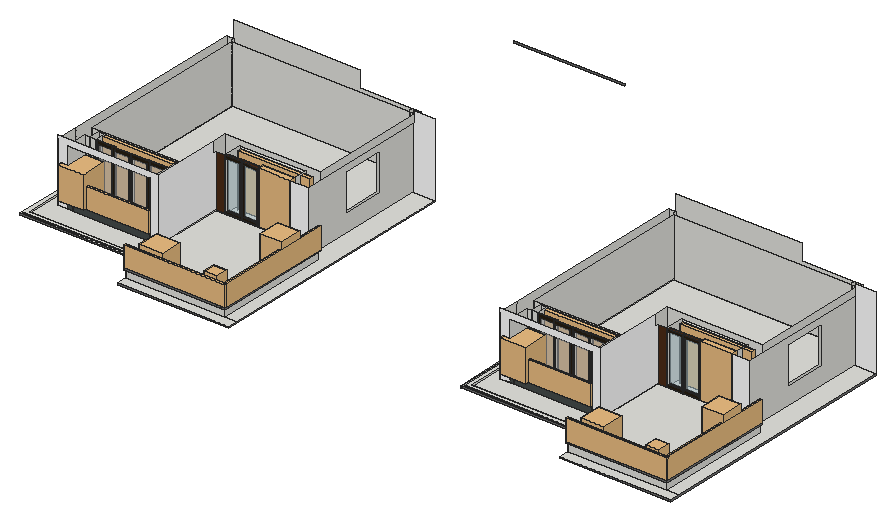
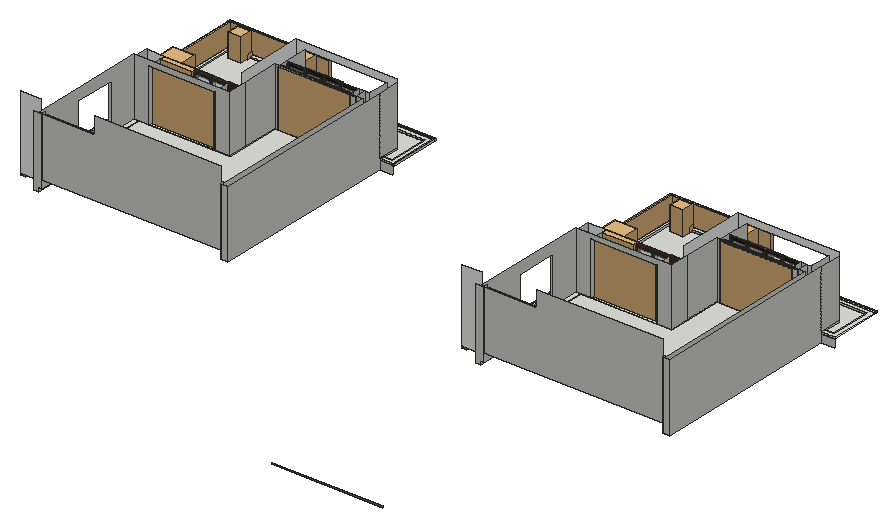
# SketchUp Ruby script. Lengths in inches.
U = 1.inch
M = Sketchup.active_model
def pt(a) = Geom::Point3d.new(a.map { |v| v * U })
def face(e, loops, mat)
  f = e.add_face(loops[0].map { |a| pt(a) })
  loops[1..].each { |l| e.add_face(l.map { |a| pt(a) }).erase! }
  f.material = f.back_material = mat if mat
  f
end
# faces: each face lists its corners as indices into pts; further lists are holes
def faces(e, pts, list, mat = nil) = list.each { |f| face(e, (f[0].is_a?(Array) ? f : [f]).map { |l| l.map { |i| pts[i] } }, mat) }
# xy, xz, yz: faces in a plane at the given z, y or x. An outline is a flat list of corners, or four numbers for a rectangle; further outlines are holes
def ring(l) = l.size == 4 ? [[l[0], l[1]], [l[2], l[1]], [l[2], l[3]], [l[0], l[3]]] : l.each_slice(2).to_a
def flat(e, list, mat, &to3) = list.each { |f| face(e, (f[0].is_a?(Array) ? f : [f]).map { |l| ring(l).map { |u, v| to3.(u, v) } }, mat) }
def xy(e, z, list, mat = nil) = flat(e, list, mat) { |x, y| [x, y, z] }
def xz(e, y, list, mat = nil) = flat(e, list, mat) { |x, z| [x, y, z] }
def yz(e, x, list, mat = nil) = flat(e, list, mat) { |y, z| [x, y, z] }
def lines(e, pts, list) = list.each { |a, b| e.add_line(pt(pts[a]), pt(pts[b])) }
# prism: a flat outline (further loops are holes) pulled along v
def prism(e, loops, v, mat = nil)
  f = face(e, loops, mat); d = Geom::Vector3d.new(v.map { |x| x * U })
  f.pushpull(f.normal.samedirection?(d) ? d.length : -d.length)
end
def box(e, o, s, mat = nil) = prism(e, [[o, [o[0] + s[0], o[1], o[2]], [o[0] + s[0], o[1] + s[1], o[2]], [o[0], o[1] + s[1], o[2]]]], [0, 0, s[2]], mat)
def at(x, y, z, deg = 0) = Geom::Transformation.translation(pt([x, y, z])) * Geom::Transformation.rotation(ORIGIN, Z_AXIS, deg.degrees)
def axes(o, x, y, z) = Geom::Transformation.new([*x, 0, *y, 0, *z, 0, *pt(o).to_a, 1])
def part(name) = M.definitions.add(name)
# library, detail: a bought-in or finely detailed component or shape, given as its bounding box
def library(name, o, s) = part(name).tap { |d| box(d.entities, o, s) }
def detail(e, o, s) = box(e.add_group.entities, o, s)
def put(e, d, t, mat = nil) = e.add_instance(d, t).tap { |i| i.material = mat if mat }
def group(e, t, mat = nil) = e.add_group.tap { |g| g.transformation = t; g.material = mat if mat }.entities
root = M.entities
M.materials.add("[Color M00]").color = [255, 255, 255]
M.materials.add("[Color M05]").color = [114, 114, 114]
M.materials.add("[Slate]").color = [70, 76, 75]
M.materials.add("[Translucent Glass Gray]2").color = [201, 201, 201]
M.materials["[Translucent Glass Gray]2"].alpha = 0.5
M.materials.add("[Translucent Glass Safety]").color = [204, 235, 244]
M.materials["[Translucent Glass Safety]"].alpha = 0.5
M.materials.add("[Wood Veneer 01]").color = [76, 44, 23]
M.materials.add("oak swatch").color = [40, 31, 19]
c1 = library("Glass Railing",[0,0,0],[139.5,4.76,42])
c2 = library("Plant",[0,0,0],[12.59,12.59,14.16])
c3 = library("plant1",[-367.84,-375.82,-125.45],[750.59,696.16,1346.74])
c4 = part("skp4FF")
put(c4.entities,c3,at(0,0,0))
c5 = library("Flora+17",[-57.52,158.6,-38.64],[66.99,62.88,77.28])
c6 = library("plant (1)",[-35.72,-28.42,0],[66.31,67.39,84.38])
c7 = part("Group\#6")
box(c7.entities,[0,0,0],[1.77,4.72,80.31],"oak swatch")
c8 = part("Exterior Sliding Doors")
xy(c8.entities,0,[[1.77,33.07,3.54,70.87],[1.77,70.87,3.54,108.66]])
xy(c8.entities,0,[[0,0,1.77,33.07],[0,108.66,1.77,141.73]],"oak swatch")
xy(c8.entities,4.72,[[0,4.72,1.77,33.07],[1.77,37.8,3.54,66.14],[1.77,75.88,3.54,103.9375],[0,108.66,1.77,137.01]],"oak swatch")
xy(c8.entities,75.59,[[1.77,37.8,3.54,66.14],[1.77,75.88,3.54,103.9375]])
xy(c8.entities,75.59,[[0,4.72,1.77,33.07],[0,108.66,1.77,137.01]],"oak swatch")
xy(c8.entities,80.31,[[0,0,1.77,33.07],[1.77,33.07,3.54,70.87],[1.77,70.87,3.54,108.66],[0,108.66,1.77,141.73]],"oak swatch")
xz(c8.entities,0,[[0,0,1.77,80.31]],"oak swatch")
xz(c8.entities,4.72,[[0,4.72,1.77,75.59]],"oak swatch")
xz(c8.entities,33.07,[[0,0,1.77,4.72],[1.77,0,3.54,80.31],[0,75.59,1.77,80.31]],"oak swatch")
xz(c8.entities,37.8,[[1.77,4.72,3.54,75.59]])
xz(c8.entities,66.14,[[1.77,4.72,3.54,75.59]],"oak swatch")
xz(c8.entities,70.87,[[1.77,0,3.54,80.31]])
xz(c8.entities,75.88,[[1.77,4.72,3.54,75.59]])
xz(c8.entities,103.9375,[[1.77,4.72,3.54,75.59]],"oak swatch")
xz(c8.entities,108.66,[[1.77,4.72,3.54,75.59]])
xz(c8.entities,108.66,[[0,0,3.54,4.72],[0,75.59,3.54,80.31]],"oak swatch")
xz(c8.entities,137.01,[[0,4.72,1.77,75.59]],"oak swatch")
xz(c8.entities,141.73,[[0,0,1.77,80.31]],"oak swatch")
yz(c8.entities,0,[[0,0,33.07,0,33.07,4.72,4.72,4.72,4.72,75.59,33.07,75.59,33.07,80.31,0,80.31],[108.66,0,141.73,0,141.73,80.31,108.66,80.31,108.66,75.59,137.01,75.59,137.01,4.72,108.66,4.72]],"oak swatch")
yz(c8.entities,1.77,[[4.72,4.72,33.07,75.59],[37.8,4.72,66.14,75.59],[75.88,4.72,103.9375,75.59],[108.66,4.72,137.01,75.59]],"[Translucent Glass Gray]2")
yz(c8.entities,1.77,[[0,0,33.07,0,33.07,4.72,4.72,4.72,4.72,75.59,33.07,75.59,33.07,80.31,0,80.31],[[33.07,0,70.87,80.31],[37.8,4.72,66.14,75.59]],[[70.87,0,141.73,80.31],[108.66,4.72,137.01,75.59],[75.88,4.72,103.9375,75.59]]],"oak swatch")
yz(c8.entities,3.54,[[[33.07,0,70.87,80.31],[37.8,4.72,66.14,75.59]],[[70.87,0,108.66,80.31],[75.88,4.72,103.9375,75.59]]],"oak swatch")
put(c8.entities,c7,at(0,33.07,0))
put(c8.entities,c7,at(0,103.9375,0))
c9 = library("Group\#21",[-0.5,-0.5,-0.1],[115.36,88.99,0.2])
c10 = library("Curtains",[0,0,0],[121.73,8.19,117.22])
c11 = part("Group\#4")
g1 = group(c11.entities,at(0,0,0))
xy(g1,0,[[0,0,6,48]],"[Wood Veneer 01]")
xy(g1,4,[[0,4,1.8125,44],[1.8125,4,6,44]])
xy(g1,80,[[0,4,1.8125,44],[1.8125,4,6,44]])
xy(g1,84,[[0,0,6,48]],"[Wood Veneer 01]")
xz(g1,0,[[0,0,6,84]],"[Wood Veneer 01]")
xz(g1,4,[[0,4,1.8125,80],[1.8125,4,6,80]])
xz(g1,44,[[0,4,1.8125,80],[1.8125,4,6,80]])
xz(g1,48,[[0,0,6,84]],"[Wood Veneer 01]")
yz(g1,0,[[[0,0,48,84],[4,4,44,80]]],"[Wood Veneer 01]")
yz(g1,1.8125,[[4,4,44,80]],"[Translucent Glass Safety]")
yz(g1,6,[[[0,0,48,84],[4,4,44,80]]],"oak swatch")
g2 = group(c11.entities,at(0,48,0),"oak swatch")
xy(g2,0,[[0,0,6,48]],"[Wood Veneer 01]")
xy(g2,4,[[0,4,1.8125,44],[1.8125,4,6,44]])
xy(g2,80,[[0,4,1.8125,44],[1.8125,4,6,44]])
xy(g2,84,[[0,0,6,48]],"[Wood Veneer 01]")
xz(g2,0,[[0,0,6,84]],"[Wood Veneer 01]")
xz(g2,4,[[0,4,1.8125,80],[1.8125,4,6,80]])
xz(g2,44,[[0,4,1.8125,80],[1.8125,4,6,80]])
xz(g2,48,[[0,0,6,84]],"[Wood Veneer 01]")
yz(g2,0,[[[0,0,48,84],[4,4,44,80]]],"[Wood Veneer 01]")
yz(g2,1.8125,[[4,4,44,80]],"[Translucent Glass Safety]")
yz(g2,6,[[[0,0,48,84],[4,4,44,80]]],"oak swatch")
c12 = library("modern+door",[0,0,0],[59.06,11.8125,86.61])
xy(root,119.75,[[2097.23,636.6875,2269.48,636.6875,2269.48,735.75,2276.89,735.75,2276.89,747.5625,2456.54,747.5625,2456.54,1019,2447.32,1019,2447.32,811.54,2440.84,811.54,2440.84,774.3125,2266.54,774.3125,2266.54,645.91,2097.23,645.91],[2989.82,636.6875,3162.07,636.6875,3162.07,735.75,3169.48,735.75,3169.48,747.5625,3349.13,747.5625,3349.13,1019,3339.91,1019,3339.91,811.54,3333.43,811.54,3333.43,774.3125,3159.13,774.3125,3159.13,645.91,2989.82,645.91]])
xy(root,122.875,[[2276.89,479.5,2500.29,488.8125],[3169.48,479.5,3392.88,488.8125],[2489.98,488.8125,2500.29,999.35],[3382.57,488.8125,3392.88,999.35]],"[Color M05]")
xy(root,126,[[2276.89,479.5,2500.29,499.9375],[3169.48,479.5,3392.88,499.9375],[2276.89,499.9375,2475.98,536.1875],[2475.98,499.9375,2500.29,499.9375,2500.29,999.35,2456.54,999.35,2456.54,735.75,2475.98,735.75],[3169.48,499.9375,3368.57,536.1875],
  [3368.57,499.9375,3392.88,499.9375,3392.88,999.35,3349.13,999.35,3349.13,735.75,3368.57,735.75],[2276.89,536.1875,2475.98,636.6875],[3169.48,536.1875,3368.57,636.6875],[2064.92,636.6875,2064.92,1019,2079.65,1019,2079.65,660.21,2097.23,660.21,2097.23,636.6875],[2276.89,636.6875,2475.98,735.75],
  [2957.51,636.6875,2957.51,1019,2972.24,1019,2972.24,660.21,2989.82,660.21,2989.82,636.6875],[3169.48,636.6875,3368.57,735.75],[2097.23,645.91,2097.23,660.21,2256.86,660.21,2256.86,774.3125,2266.54,774.3125,2266.54,645.91],[2989.82,645.91,2989.82,660.21,3149.44,660.21,3149.44,774.3125,3159.13,774.3125,3159.13,645.91],[2276.89,735.75,2456.54,747.5625],
  [3169.48,735.75,3349.13,747.5625],[2440.84,811.54,2447.32,1019],[3333.43,811.54,3339.91,1019]])
xy(root,142.875,[[2276.89,495.25,2475.98,499.9375],[2475.98,495.25,2480.67,499.9375],[3169.48,495.25,3368.57,499.9375],[3368.57,495.25,3373.26,499.9375],[2276.89,499.9375,2276.89,536.1875,2037.92,536.1875,2037.92,636.6875,2064.92,636.6875,2064.92,628.3125,2046.17,628.3125,2046.17,544.8125,2283.23,544.8125,2283.23,507.75,2469.67,507.75,2469.67,721.95,2456.54,721.95,2456.54,735.75,2475.98,735.75,2475.98,499.9375],
  [2475.98,499.9375,2480.67,735.75],[3169.48,499.9375,3169.48,536.1875,2930.51,536.1875,2930.51,636.6875,2957.51,636.6875,2957.51,628.3125,2938.76,628.3125,2938.76,544.8125,3175.82,544.8125,3175.82,507.75,3362.26,507.75,3362.26,721.95,3349.13,721.95,3349.13,735.75,3368.57,735.75,3368.57,499.9375],[3368.57,499.9375,3373.26,735.75],[2283.23,507.75,2469.67,507.75,2469.67,721.95,2456.54,721.95,2456.54,735.75,2269.48,735.75,2269.48,592.75,2064.92,592.75,2064.92,628.3125,2046.17,628.3125,2046.17,544.8125,2283.23,544.8125],[3175.82,507.75,3362.26,507.75,3362.26,721.95,3349.13,721.95,3349.13,735.75,3162.07,735.75,3162.07,592.75,2957.51,592.75,2957.51,628.3125,2938.76,628.3125,2938.76,544.8125,3175.82,544.8125],
  [2037.92,531.5,2276.89,536.1875],[2927.19,531.5,2930.51,536.1875],[2930.51,531.5,3169.48,536.1875],[2927.19,536.1875,2930.32,636.6875],[2930.32,536.1875,2930.51,636.6875],
  [2064.92,592.75,2094.14,592.75,2094.14,604.1,2084.76,604.1,2084.76,636.6875,2064.92,636.6875],[2251.32,592.75,2269.48,636.6875],[2957.51,592.75,2986.73,592.75,2986.73,604.1,2977.35,604.1,2977.35,636.6875,2957.51,636.6875],[3143.91,592.75,3162.07,636.6875],[2084.76,604.1,2251.32,636.6875],
  [2977.35,604.1,3143.91,636.6875],[2094.14,636.6875,2106.51,660.21],[2106.51,636.6875,2251.32,660.21],[2986.73,636.6875,2999.1,660.21],[2999.1,636.6875,3143.91,660.21],
  [2079.65,660.21,2256.86,660.21,2256.86,774.3125,2440.84,774.3125,2440.84,1012.63,2079.65,1012.63],[2972.24,660.21,3149.44,660.21,3149.44,774.3125,3333.43,774.3125,3333.43,1012.63,2972.24,1012.63],[2287.52,735.75,2419.84,774.3125],[3180.11,735.75,3312.43,774.3125],[2440.84,774.3125,2450.84,1012.63],
  [3333.43,774.3125,3343.43,1012.63],[2079.65,1012.63,2440.84,1019],[2972.24,1012.63,3333.43,1019]])
xy(root,146.125,[[2276.89,495.25,2480.67,495.25,2480.67,735.75,2475.98,735.75,2475.98,499.9375,2276.89,499.9375],[3169.48,495.25,3373.26,495.25,3373.26,735.75,3368.57,735.75,3368.57,499.9375,3169.48,499.9375],[2276.89,499.9375,2475.98,499.9375,2475.98,735.75,2456.54,735.75,2456.54,721.95,2469.67,721.95,2469.67,507.75,2283.23,507.75,2283.23,544.8125,2046.17,544.8125,2046.17,628.3125,2064.92,628.3125,2064.92,636.6875,2037.92,636.6875,2037.92,536.1875,2276.89,536.1875],[3169.48,499.9375,3368.57,499.9375,3368.57,735.75,3349.13,735.75,3349.13,721.95,3362.26,721.95,3362.26,507.75,3175.82,507.75,3175.82,544.8125,2938.76,544.8125,2938.76,628.3125,2957.51,628.3125,2957.51,636.6875,2930.51,636.6875,2930.51,536.1875,3169.48,536.1875],[2037.92,531.5,2276.89,536.1875],
  [2927.19,531.5,2930.51,536.1875],[2930.51,531.5,3169.48,536.1875],[2927.19,536.1875,2930.32,636.6875],[2930.32,536.1875,2930.51,636.6875]])
xy(root,156.6875,[[2084.76,592.75,2094.14,604.1],[2094.14,592.75,2251.32,604.1],[2977.35,592.75,2986.73,604.1],[2986.73,592.75,3143.91,604.1]],"[Slate]")
xz(root,479.5,[[2276.89,122.875,2500.29,126],[3169.48,122.875,3392.88,126]],"[Color M05]")
xz(root,495.25,[[2276.89,142.875,2480.67,146.125],[3169.48,142.875,3373.26,146.125]],"[Color M05]")
xz(root,499.9375,[[2276.89,126,2475.98,142.875],[3169.48,126,3368.57,142.875],[2276.89,142.875,2475.98,146.125],[3169.48,142.875,3368.57,146.125]])
xz(root,507.75,[[2283.23,142.875,2469.67,146.125],[3175.82,142.875,3362.26,146.125]])
xz(root,531.5,[[2927.19,142.875,2930.51,146.125]])
xz(root,531.5,[[2037.92,142.875,2276.89,146.125],[2930.51,142.875,3169.48,146.125]],"[Color M05]")
xz(root,536.1875,[[2037.92,142.875,2276.89,146.125],[2927.19,142.875,2930.32,146.125],[2930.32,142.875,2930.51,146.125],[2930.51,142.875,3169.48,146.125]])
xz(root,544.8125,[[2046.17,142.875,2283.23,146.125],[2938.76,142.875,3175.82,146.125]])
xz(root,592.75,[[2064.92,142.875,2084.76,142.875,2084.76,257.1875,2251.32,257.1875,2251.32,142.875,2269.48,142.875,2269.48,270.375,2064.92,270.375],[2957.51,142.875,2977.35,142.875,2977.35,257.1875,3143.91,257.1875,3143.91,142.875,3162.07,142.875,3162.07,270.375,2957.51,270.375]],"[Color M00]")
xz(root,592.75,[[2084.76,142.875,2094.14,156.6875],[2094.14,142.875,2251.32,156.6875],[2977.35,142.875,2986.73,156.6875],[2986.73,142.875,3143.91,156.6875]],"[Slate]")
xz(root,604.1,[[2084.76,142.875,2094.14,156.6875],[2094.14,142.875,2251.32,156.6875],[2977.35,142.875,2986.73,156.6875],[2986.73,142.875,3143.91,156.6875]])
xz(root,628.3125,[[2046.17,142.875,2064.92,146.125],[2938.76,142.875,2957.51,146.125]])
xz(root,636.6875,[[2097.23,119.75,2269.48,119.75,2269.48,142.875,2064.92,142.875,2064.92,126,2097.23,126],[2989.82,119.75,3162.07,119.75,3162.07,142.875,2957.51,142.875,2957.51,126,2989.82,126],[2037.92,126,2064.92,142.875],[2930.51,126,2957.51,142.875],[2037.92,142.875,2064.92,146.125],
  [2084.76,142.875,2094.14,257.1875],[2094.14,142.875,2106.51,257.1875],[2927.19,142.875,2930.32,146.125],[2930.32,142.875,2930.51,146.125],[2930.51,142.875,2957.51,146.125],
  [2977.35,142.875,2986.73,257.1875],[2986.73,142.875,2999.1,257.1875]])
xz(root,645.91,[[2097.23,119.75,2266.54,126],[2989.82,119.75,3159.13,126]])
xz(root,660.21,[[2079.65,126,2256.86,142.875],[2972.24,126,3149.44,142.875],[2079.65,142.875,2079.65,259.3125,2256.86,259.3125,2256.86,142.875,2251.32,142.875,2251.32,257.1875,2094.14,257.1875,2094.14,142.875],[2094.14,142.875,2106.51,257.1875],[2972.24,142.875,2972.24,259.3125,3149.44,259.3125,3149.44,142.875,3143.91,142.875,3143.91,257.1875,2986.73,257.1875,2986.73,142.875],
  [2986.73,142.875,2999.1,257.1875]])
xz(root,721.95,[[2456.54,142.875,2469.67,146.125],[3349.13,142.875,3362.26,146.125]])
xz(root,735.75,[[2269.48,119.75,2276.89,119.75,2276.89,126,2456.54,126,2456.54,142.875,2269.48,142.875],[3162.07,119.75,3169.48,119.75,3169.48,126,3349.13,126,3349.13,142.875,3162.07,142.875],[2456.54,126,2475.98,142.875],[3349.13,126,3368.57,142.875],[2456.54,142.875,2475.98,146.125],
  [2475.98,142.875,2480.67,146.125],[3349.13,142.875,3368.57,146.125],[3368.57,142.875,3373.26,146.125]])
xz(root,735.75,[[2419.84,142.875,2456.54,249.4375],[3312.43,142.875,3349.13,249.4375]],"[Color M00]")
xz(root,735.75,[[2269.48,142.875,2287.52,249.4375],[3162.07,142.875,3180.11,249.4375]],"[Wood Veneer 01]")
xz(root,747.5625,[[2276.89,119.75,2456.54,126],[3169.48,119.75,3349.13,126]])
xz(root,774.3125,[[2266.54,119.75,2440.84,119.75,2440.84,142.875,2256.86,142.875,2256.86,126,2266.54,126],[3159.13,119.75,3333.43,119.75,3333.43,142.875,3149.44,142.875,3149.44,126,3159.13,126],[2256.86,142.875,2256.86,259.3125,2450.84,259.3125,2450.84,142.875,2419.84,142.875,2419.84,249.4375,2287.52,249.4375,2287.52,142.875],[3149.44,142.875,3149.44,259.3125,3343.43,259.3125,3343.43,142.875,3312.43,142.875,3312.43,249.4375,3180.11,249.4375,3180.11,142.875]])
xz(root,811.54,[[2440.84,119.75,2447.32,126],[3333.43,119.75,3339.91,126]])
xz(root,999.35,[[2456.54,126,2500.29,126,2500.29,274.0625,2459.67,274.0625,2459.67,249.4375,2456.54,249.4375],[3349.13,126,3392.88,126,3392.88,274.0625,3352.26,274.0625,3352.26,249.4375,3349.13,249.4375]],"[Color M00]")
xz(root,1012.63,[[2079.65,142.875,2440.84,259.3125],[2440.84,142.875,2450.84,259.3125],[2972.24,142.875,3333.43,259.3125],[3333.43,142.875,3343.43,259.3125]])
xz(root,1019,[[2447.32,119.75,2447.32,126,2440.84,126,2440.84,262.875,2456.54,262.875,2456.54,119.75],[3339.91,119.75,3339.91,126,3333.43,126,3333.43,262.875,3349.13,262.875,3349.13,119.75],[2064.92,126,2079.65,262.875],[2957.51,126,2972.24,262.875],[2079.65,142.875,2079.65,295.8125,2333.29,295.8125,2333.29,262.875,2440.84,262.875,2440.84,142.875],
  [2972.24,142.875,2972.24,295.8125,3225.88,295.8125,3225.88,262.875,3333.43,262.875,3333.43,142.875]])
xz(root,1478.85,[[2276.89,122.875,2500.29,126]],"[Color M05]")
yz(root,2046.17,[[544.8125,142.875,628.3125,146.125]])
yz(root,2064.92,[[636.6875,126,1019,262.875],[592.75,142.875,628.3125,146.125],[628.3125,142.875,636.6875,146.125],[592.75,146.125,636.6875,262.875]])
yz(root,2079.65,[[660.21,126,1019,142.875],[660.21,142.875,1012.63,259.3125],[1012.63,142.875,1019,262.875]])
yz(root,2084.76,[[604.1,142.875,636.6875,142.875,636.6875,257.1875,592.75,257.1875,592.75,156.6875,604.1,156.6875]])
yz(root,2094.14,[[592.75,142.875,604.1,156.6875],[636.6875,142.875,660.21,257.1875]])
yz(root,2097.23,[[636.6875,119.75,645.91,126]])
yz(root,2106.51,[[636.6875,142.875,660.21,257.1875]])
yz(root,2251.32,[[592.75,142.875,604.1,156.6875],[604.1,142.875,604.1,156.6875,592.75,156.6875,592.75,257.1875,636.6875,257.1875,636.6875,142.875],[636.6875,142.875,660.21,257.1875]])
yz(root,2256.86,[[660.21,126,735.75,142.875],[735.75,126,774.3125,142.875],[660.21,142.875,735.75,259.3125],[735.75,142.875,774.3125,259.3125]])
yz(root,2266.54,[[645.91,119.75,774.3125,126]])
yz(root,2269.48,[[636.6875,119.75,735.75,142.875]])
yz(root,2269.48,[[592.75,142.875,735.75,142.875,735.75,249.4375,728.9375,249.4375,728.9375,270.375,592.75,270.375]],"[Color M00]")
yz(root,2276.89,[[735.75,119.75,747.5625,126],[499.9375,126,536.1875,142.875],[495.25,142.875,499.9375,146.125],[499.9375,142.875,531.5,146.125],[531.5,142.875,536.1875,146.125]])
yz(root,2283.23,[[507.75,142.875,544.8125,146.125]])
yz(root,2287.52,[[735.75,142.875,774.3125,249.4375]])
yz(root,2419.84,[[735.75,142.875,774.3125,249.4375]])
yz(root,2440.84,[[774.3125,119.75,811.54,119.75,811.54,126,1019,126,1019,142.875,774.3125,142.875],[1012.63,142.875,1019,262.875]])
yz(root,2447.32,[[811.54,119.75,1019,126]])
yz(root,2450.84,[[[774.3125,142.875,1012.63,259.3125],[831.26,160.58,916.82,236.83]]])
yz(root,2456.54,[[[735.75,126,999.35,249.4375],[831.26,160.58,916.82,236.83]],[721.95,142.875,735.75,146.125]])
yz(root,2469.67,[[507.75,142.875,721.95,146.125]])
yz(root,2475.98,[[499.9375,126,735.75,142.875],[499.9375,142.875,735.75,146.125]])
yz(root,2480.67,[[495.25,142.875,735.75,146.125]],"[Color M05]")
yz(root,2500.29,[[479.5,122.875,999.35,126]],"[Color M05]")
yz(root,2927.19,[[531.5,142.875,536.1875,146.125],[536.1875,142.875,636.6875,146.125]])
yz(root,2930.32,[[536.1875,142.875,636.6875,146.125]])
yz(root,2930.51,[[531.5,142.875,536.1875,146.125],[536.1875,142.875,636.6875,146.125]])
yz(root,2938.76,[[544.8125,142.875,628.3125,146.125]])
yz(root,2957.51,[[636.6875,126,1019,262.875],[592.75,142.875,628.3125,146.125],[628.3125,142.875,636.6875,146.125],[592.75,146.125,636.6875,262.875]])
yz(root,2972.24,[[660.21,126,1019,142.875],[660.21,142.875,1012.63,259.3125],[1012.63,142.875,1019,262.875]])
yz(root,2977.35,[[604.1,142.875,636.6875,142.875,636.6875,257.1875,592.75,257.1875,592.75,156.6875,604.1,156.6875]])
yz(root,2986.73,[[592.75,142.875,604.1,156.6875],[636.6875,142.875,660.21,257.1875]])
yz(root,2989.82,[[636.6875,119.75,645.91,126]])
yz(root,2999.1,[[636.6875,142.875,660.21,257.1875]])
yz(root,3143.91,[[592.75,142.875,604.1,156.6875],[604.1,142.875,604.1,156.6875,592.75,156.6875,592.75,257.1875,636.6875,257.1875,636.6875,142.875],[636.6875,142.875,660.21,257.1875]])
yz(root,3149.44,[[660.21,126,735.75,142.875],[735.75,126,774.3125,142.875],[660.21,142.875,735.75,259.3125],[735.75,142.875,774.3125,259.3125]])
yz(root,3159.13,[[645.91,119.75,774.3125,126]])
yz(root,3162.07,[[636.6875,119.75,735.75,142.875]])
yz(root,3162.07,[[592.75,142.875,735.75,142.875,735.75,249.4375,728.9375,249.4375,728.9375,270.375,592.75,270.375]],"[Color M00]")
yz(root,3169.48,[[735.75,119.75,747.5625,126],[499.9375,126,536.1875,142.875],[495.25,142.875,499.9375,146.125],[499.9375,142.875,531.5,146.125],[531.5,142.875,536.1875,146.125]])
yz(root,3175.82,[[507.75,142.875,544.8125,146.125]])
yz(root,3180.11,[[735.75,142.875,774.3125,249.4375]])
yz(root,3312.43,[[735.75,142.875,774.3125,249.4375]])
yz(root,3333.43,[[774.3125,119.75,811.54,119.75,811.54,126,1019,126,1019,142.875,774.3125,142.875],[1012.63,142.875,1019,262.875]])
yz(root,3339.91,[[811.54,119.75,1019,126]])
yz(root,3343.43,[[[774.3125,142.875,1012.63,259.3125],[831.26,160.58,916.82,236.83]]])
yz(root,3349.13,[[[735.75,126,999.35,249.4375],[831.26,160.58,916.82,236.83]],[721.95,142.875,735.75,146.125]])
yz(root,3362.26,[[507.75,142.875,721.95,146.125]])
yz(root,3368.57,[[499.9375,126,735.75,142.875],[499.9375,142.875,735.75,146.125]])
yz(root,3373.26,[[495.25,142.875,735.75,146.125]],"[Color M05]")
yz(root,3392.88,[[479.5,122.875,999.35,126]],"[Color M05]")
put(root,c1,axes([3169.59,495.25,146.125],[1.46,0,0],[0,1,0],[0,0,1]))
put(root,c1,axes([2277,495.25,146.125],[1.46,0,0],[0,1,0],[0,0,1]))
put(root,c2,axes([3322.12,504.29,142.875],[0.7,0,0],[0,0.7,0],[0,0,0.7]))
put(root,c2,axes([2429.53,504.29,142.875],[0.7,0,0],[0,0.7,0],[0,0,0.7]))
put(root,c4,axes([3335.6,518.07,147.31],[0.03534,0,0],[0,0.03534,0],[0,0,0.03534]))
put(root,c4,axes([2443.01,518.07,147.31],[0.03534,0,0],[0,0.03534,0],[0,0,0.03534]))
put(root,c2,axes([3186.16,515.77,142.875],[0.7,0,0],[0,0.7,0],[0,0,0.7]))
put(root,c2,axes([2293.57,515.77,142.875],[0.7,0,0],[0,0.7,0],[0,0,0.7]))
put(root,c5,axes([3232.35,392.03,165.58],[0.71,0,0],[0,0.71,0],[0,0,0.71]))
put(root,c5,axes([2339.76,392.03,165.58],[0.71,0,0],[0,0.71,0],[0,0,0.71]))
put(root,c1,axes([2977.35,589.78,157.48],[1.194,0,0],[0,1,0],[0,0,1]))
put(root,c1,axes([2084.76,589.78,157.48],[1.194,0,0],[0,1,0],[0,0,1]))
put(root,c6,axes([2992.63,605.83,158.18],[0.77,0,0],[0,0.77,0],[0,0,0.77]))
put(root,c6,axes([2100.04,605.83,158.18],[0.77,0,0],[0,0.77,0],[0,0,0.77]))
put(root,c1,axes([3373.33,498.26,146.09],[0,1.70244,0],[-1,0,0],[0,0,1]))
put(root,c1,axes([2480.74,498.26,146.09],[0,1.70244,0],[-1,0,0],[0,0,1]))
put(root,c8,axes([3000.08,638.46,142.875],[0,-1,0],[0.99858,0,0],[0,0,1.4151]))
put(root,c8,axes([2107.49,638.46,142.875],[0,-1,0],[0.99858,0,0],[0,0,1.4151]))
put(root,c9,at(3208.3,595.88,119.375))
put(root,c9,at(2315.71,595.88,119.375))
put(root,c10,axes([2998.5625,652.02,142.875],[1.19408,0,0],[0,1,0],[0,0,0.96546]))
put(root,c10,axes([2105.97,652.02,142.875],[1.19408,0,0],[0,1,0],[0,0,0.96546]))
put(root,c6,axes([3352.77,656.78,146.125],[0.67,0,0],[0,0.67,0],[0,0,0.67]))
put(root,c6,axes([2460.18,656.78,146.125],[0.67,0,0],[0,0.67,0],[0,0,0.67]))
put(root,c11,axes([3179.59,741.75,142.875],[0,-1,0],[0.71,0,0],[0,0,1.26]))
put(root,c11,axes([2287,741.75,142.875],[0,-1,0],[0.71,0,0],[0,0,1.26]))
put(root,c12,axes([3248.06,735.75,142.875],[1.09,0,0],[0,1,0],[0,0,1.23031]))
put(root,c12,axes([2355.47,735.75,142.875],[1.09,0,0],[0,1,0],[0,0,1.23031]))
put(root,c10,axes([3187.16,760.24,135.21],[1.19408,0,0],[0,1,0],[0,0,0.96546]))
put(root,c10,axes([2294.57,760.24,135.21],[1.19408,0,0],[0,1,0],[0,0,0.96546]))
